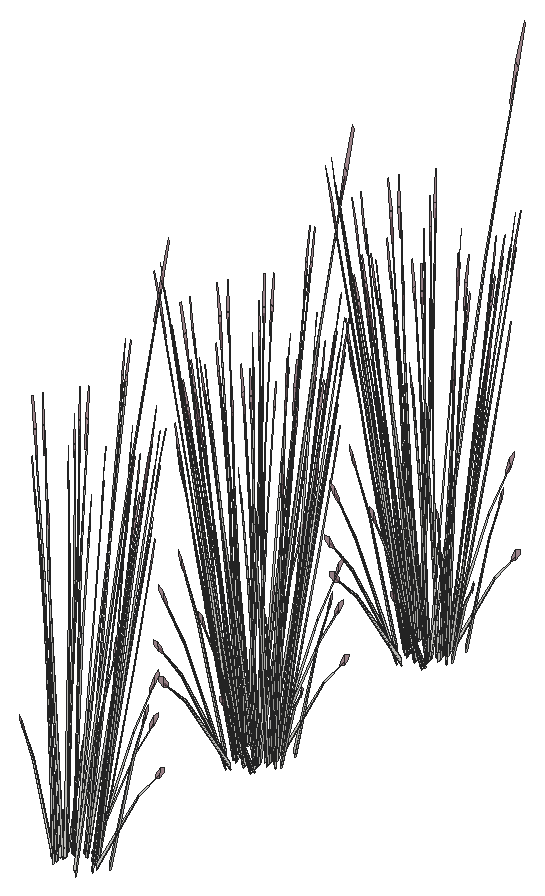
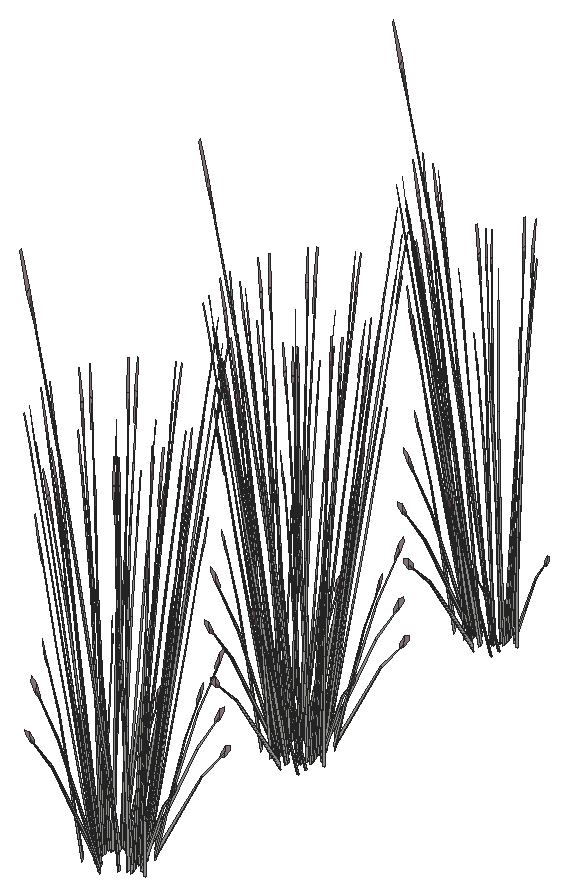
# SketchUp Ruby script. Lengths in inches.
U = 1.inch
M = Sketchup.active_model
def pt(a) = Geom::Point3d.new(a.map { |v| v * U })
def face(e, loops, mat)
  f = e.add_face(loops[0].map { |a| pt(a) })
  loops[1..].each { |l| e.add_face(l.map { |a| pt(a) }).erase! }
  f.material = f.back_material = mat if mat
  f
end
# faces: each face lists its corners as indices into pts; further lists are holes
def faces(e, pts, list, mat = nil) = list.each { |f| face(e, (f[0].is_a?(Array) ? f : [f]).map { |l| l.map { |i| pts[i] } }, mat) }
# xy, xz, yz: faces in a plane at the given z, y or x. An outline is a flat list of corners, or four numbers for a rectangle; further outlines are holes
def ring(l) = l.size == 4 ? [[l[0], l[1]], [l[2], l[1]], [l[2], l[3]], [l[0], l[3]]] : l.each_slice(2).to_a
def flat(e, list, mat, &to3) = list.each { |f| face(e, (f[0].is_a?(Array) ? f : [f]).map { |l| ring(l).map { |u, v| to3.(u, v) } }, mat) }
def xy(e, z, list, mat = nil) = flat(e, list, mat) { |x, y| [x, y, z] }
def xz(e, y, list, mat = nil) = flat(e, list, mat) { |x, z| [x, y, z] }
def yz(e, x, list, mat = nil) = flat(e, list, mat) { |y, z| [x, y, z] }
def lines(e, pts, list) = list.each { |a, b| e.add_line(pt(pts[a]), pt(pts[b])) }
# prism: a flat outline (further loops are holes) pulled along v
def prism(e, loops, v, mat = nil)
  f = face(e, loops, mat); d = Geom::Vector3d.new(v.map { |x| x * U })
  f.pushpull(f.normal.samedirection?(d) ? d.length : -d.length)
end
def box(e, o, s, mat = nil) = prism(e, [[o, [o[0] + s[0], o[1], o[2]], [o[0] + s[0], o[1] + s[1], o[2]], [o[0], o[1] + s[1], o[2]]]], [0, 0, s[2]], mat)
def at(x, y, z, deg = 0) = Geom::Transformation.translation(pt([x, y, z])) * Geom::Transformation.rotation(ORIGIN, Z_AXIS, deg.degrees)
def axes(o, x, y, z) = Geom::Transformation.new([*x, 0, *y, 0, *z, 0, *pt(o).to_a, 1])
def part(name) = M.definitions.add(name)
# library, detail: a bought-in or finely detailed component or shape, given as its bounding box
def library(name, o, s) = part(name).tap { |d| box(d.entities, o, s) }
def detail(e, o, s) = box(e.add_group.entities, o, s)
def put(e, d, t, mat = nil) = e.add_instance(d, t).tap { |i| i.material = mat if mat }
def group(e, t, mat = nil) = e.add_group.tap { |g| g.transformation = t; g.material = mat if mat }.entities
root = M.entities
M.materials.add("LightPink_Translucent").color = [144, 107, 117]
M.materials["LightPink_Translucent"].alpha = 0.75
c1 = part("blade")
p = [[2.15,0.21,22],[0,0.17,0],[0.09,0.45,0],[2.18,0.31,22],[2.29,0.31,22],[0.38,0.45,0],
  [2.48,0.24,33],[2.49,0.24,33],[2.48,0.22,33]]
faces(c1.entities,p,[[0,1,2,3],[4,5,2,3],[6,3,4,7],[8,0,3,6]])
c2 = part("seeds")
p = [[0.3,-0.1,1.38],[-0.01,-0.03,1.59],[-0.01,-0.03,0.03],[0.14,-0.07,-0.07],[0.29,-0.03,3],[0.15,0.01,3.11]]
faces(c2.entities,p,[[0,1,2,3],[1,0,4,5]],"LightPink_Translucent")
c3 = part("blade with seeds")
put(c3.entities,c1,at(0,0,0))
put(c3.entities,c2,axes([2.4,0.25,30.99],[1.5799,-0.05474,1.17369],[-0.12525,1.92788,0.29478],[-0.07173,-0.02425,1.56792]))
put(root,c3,axes([403.71,539.25,4.73],[-0.09971,0.42522,0.48003],[-0.32782,-0.1454,0.3958],[0.12892,-0.02555,0.9933]))
put(root,c3,axes([400.64,538.56,5.05],[0.29332,0.1301,0.35414],[-0.08555,0.37955,-0.4572],[-0.11809,0.0348,0.87481]))
put(root,c3,axes([404.3,540.63,4.71],[-0.03191,-0.04083,1.77383],[0.06981,-0.43764,-0.16761],[0.12571,-0.02796,0.31391]))
put(root,c3,axes([400.14,538.85,4.72],[-0.05763,0.06055,1.74944],[0.0049,0.44239,-0.27667],[-0.13211,0.05753,0.14031]))
put(root,c3,axes([400.51,538.43,5.03],[0.17758,0.42229,-0.1216],[-0.31518,0.20752,-0.67495],[-0.13282,0.05572,1.02557]))
put(root,c3,axes([403.19,540.25,5.03],[0.0189,-0.47427,-0.1216],[0.35781,0.01296,-0.67495],[0.13781,0.03295,1.02557]))
put(root,c3,axes([403.14,540.07,5.05],[-0.20082,-0.29199,0.35414],[0.2293,-0.2764,-0.4572],[0.1165,0.04206,0.87481]))
put(root,c3,axes([403.5,539.97,4.72],[0.07571,-0.00789,1.74944],[0.20767,-0.36231,-0.27667],[0.13467,0.04783,0.14031]))
put(root,c3,axes([400.47,539.61,4.73],[-0.08753,-0.42921,0.48003],[0.34336,-0.07449,0.3958],[-0.1012,0.10094,0.9933]))
put(root,c3,axes([400.41,539.53,4.73],[-0.2423,-0.19613,0.0643],[0.14107,-0.2793,0.50621],[-0.07768,0.0903,0.77189]))
put(root,c3,axes([400.6875,539.47,5.05],[0.30722,-0.06665,0.35414],[0.08112,0.381,-0.4572],[-0.08804,0.10234,0.87481]))
put(root,c3,axes([399.5,539.3,4.71],[0.04504,0.01251,1.77383],[0.13934,0.41205,-0.16761],[-0.0922,0.10815,0.31391]))
put(root,c3,axes([403.32,540.33,4.73],[-0.01777,0.35463,0.0643],[-0.26836,-0.00972,0.50621],[0.1028,0.03711,0.77189]))
put(root,c3,axes([403.34,540.22,4.73],[-0.26024,0.30729,0.48003],[-0.22444,-0.32634,0.3958],[0.1221,0.05668,0.9933]))
put(root,c3,axes([399.99,540.55,5.65],[0.31145,0.12449,-0.06488],[-0.0958,0.38314,-0.29416],[-0.05094,0.05817,0.97024]))
put(root,c3,axes([402.52,540.57,5.05],[-0.05451,-0.37564,0.35414],[0.31161,-0.09919,-0.4572],[0.0837,0.10765,0.87481]))
put(root,c3,axes([402.72,538.41,4.47],[-0.30498,-0.24231,1.38283],[0.32203,-0.37727,0.59665],[0.0984,0.22736,1.33663]))
put(root,c3,axes([400.53,539.4375,5.03],[0.32648,0.25715,-0.1216],[-0.18809,0.3724,-0.67495],[-0.09224,0.12945,1.02557]))
put(root,c3,axes([402.49,540.77,5.03],[0.21031,-0.39918,-0.1216],[0.30457,0.22997,-0.67495],[0.10587,0.11278,1.02557]))
put(root,c3,axes([401.1,540.23,5.05],[0.23881,-0.24554,0.35414],[0.22606,0.28036,-0.4572],[-0.0344,0.14245,0.87481]))
put(root,c3,axes([402.21,541.1,4.71],[0.00104,-0.05646,1.77383],[0.30246,-0.2491,-0.16761],[0.10506,0.08891,0.31391]))
put(root,c3,axes([400.88,540.45,4.73],[-0.29004,-0.02173,0.0643],[0.00795,-0.32812,0.50621],[-0.03035,0.12569,0.77189]))
put(root,c3,axes([400.98,540.48,4.73],[-0.25132,-0.3182,0.48003],[0.2669,-0.27442,0.3958],[-0.04636,0.14929,0.9933]))
put(root,c3,axes([401.77,540.63,5.05],[0.1064,-0.35863,0.35414],[0.31043,0.1046,-0.4572],[0.02846,0.14439,0.87481]))
put(root,c3,axes([402.56,540.91,4.73],[-0.16041,0.29625,0.0643],[-0.22843,-0.17248,0.50621],[0.07385,0.09498,0.77189]))
put(root,c3,axes([402.1875,541.91,5.65],[0.2439,-0.26754,-0.06488],[0.22348,0.29302,-0.29416],[0.01573,0.08303,0.97024]))
put(root,c3,axes([402.63,540.83,4.73],[-0.35104,0.10702,0.48003],[-0.06092,-0.41983,0.3958],[0.08256,0.12373,0.9933]))
put(root,c3,axes([401.67,540.96,4.73],[-0.26007,0.1585,0.0643],[-0.12729,-0.28902,0.50621],[0.02512,0.1274,0.77189]))
put(root,c3,axes([400.15,540.51,4.72],[-0.00877,0.09229,1.74944],[0.24897,0.32105,-0.27667],[-0.06518,0.15182,0.14031]))
put(root,c3,axes([400.95,540.3,5.4],[0.3879,0.02311,-0.13498],[-0.0106,0.43749,-0.74919],[-0.02694,0.1685,1.13838]))
put(root,c3,axes([401.67,540.78,5.03],[0.34538,-0.21713,-0.1216],[0.16972,0.38536,-0.67495],[0.04557,0.16239,1.02557]))
put(root,c3,axes([401.77,540.93,5.0625],[-0.34777,-0.12192,0.53283],[0.11892,-0.40083,0.43934],[0.0209,0.15763,1.10256]))
put(root,c3,axes([400.125,541.45,4.71],[0.04004,-0.02816,1.77383],[0.33095,0.18728,-0.16761],[-0.00778,0.15594,0.31391]))
put(root,c3,axes([401.58,541.65,4.72],[0.04474,0.0751,1.74944],[0.36104,0.0295,-0.27667],[0.03631,0.16562,0.14031]))
put(root,c3,axes([401.89,557.86,4.72],[-0.05398,-0.06539,1.74944],[-0.36026,0.04145,-0.27667],[-0.0575,-0.15639,0.14031]))
put(root,c3,axes([403.51,558.66,4.72],[-0.00341,-0.09282,1.74944],[-0.28775,-0.26825,-0.27667],[0.04449,-0.16261,0.14031]))
put(root,c3,axes([403.43,558.33,4.71],[-0.03584,0.03562,1.77383],[-0.35118,-0.12018,-0.16761],[-0.01271,-0.15545,0.31391]))
put(root,c3,axes([401.52,557.64,4.71],[-0.00658,0.0559,1.77383],[-0.32474,0.20287,-0.16761],[-0.09556,-0.1037,0.31391]))
put(root,c3,axes([401.45,558.64,5.09],[0.39316,-0.11987,0.53763],[0.06823,0.47021,0.4433],[-0.09247,-0.13858,1.11249]))
put(root,c3,axes([402.34,558.72,4.73],[0.34777,0.12192,0.48003],[-0.11892,0.40083,0.3958],[-0.0209,-0.15763,0.9933]))
put(root,c3,axes([402.4375,558.87,5.03],[-0.34538,0.21713,-0.1216],[-0.16972,-0.38536,-0.67495],[-0.04557,-0.16239,1.02557]))
put(root,c3,axes([403.15,559.36,5.03],[-0.3879,-0.02311,-0.1216],[0.0106,-0.43749,-0.67495],[0.02694,-0.1685,1.02557]))
put(root,c3,axes([402.43,558.69,4.73],[0.26007,-0.1585,0.0643],[0.12729,0.28902,0.50621],[-0.02512,-0.1274,0.77189]))
put(root,c3,axes([401.54,558.74,4.73],[0.16041,-0.29625,0.0643],[0.22843,0.17248,0.50621],[-0.07385,-0.09498,0.77189]))
put(root,c3,axes([402.33,559.02,5.05],[-0.1064,0.35863,0.35414],[-0.31043,-0.1046,-0.4572],[-0.02846,-0.14439,0.87481]))
put(root,c3,axes([403.125,559.17,4.73],[0.25132,0.3182,0.48003],[-0.2669,0.27442,0.3958],[0.04636,-0.14929,0.9933]))
put(root,c3,axes([401.61,558.71,5.43],[-0.23555,0.44708,-0.13619],[-0.34112,-0.25757,-0.75594],[-0.11858,-0.12631,1.14864]))
put(root,c3,axes([403.22,559.2,4.73],[0.29004,0.02173,0.0643],[-0.00795,0.32812,0.50621],[0.03035,-0.12569,0.77189]))
put(root,c3,axes([403,559.42,5.05],[-0.23881,0.24554,0.35414],[-0.22606,-0.28036,-0.4572],[0.0344,-0.14245,0.87481]))
put(root,c3,axes([400.71,558.58,4.72],[-0.07594,-0.00329,1.74944],[-0.24177,0.32918,-0.27667],[-0.129,-0.06726,0.14031]))
put(root,c3,axes([403.58,560.22,5.03],[-0.32648,-0.25715,-0.1216],[0.18809,-0.3724,-0.67495],[0.09224,-0.12945,1.02557]))
put(root,c3,axes([401.59,559.08,5.05],[0.05451,0.37564,0.35414],[-0.31161,0.09919,-0.4572],[-0.0837,-0.10765,0.87481]))
put(root,c3,axes([400.65,559.32,5.09],[0.29147,-0.34417,0.53763],[0.25138,0.3655,0.4433],[-0.13675,-0.06349,1.11249]))
put(root,c3,axes([404.38,560.11,4.71],[-0.0461,-0.00354,1.77383],[-0.19143,-0.37951,-0.16761],[0.07688,-0.12478,0.31391]))
put(root,c3,axes([400.78,559.32,4.73],[0.01777,-0.35463,0.0643],[0.26836,0.00972,0.50621],[-0.1028,-0.03711,0.77189]))
put(root,c3,axes([403.42,560.18,5.05],[-0.30722,0.06665,0.35414],[-0.08112,-0.381,-0.4572],[0.08804,-0.10234,0.87481]))
put(root,c3,axes([403.7,560.12,4.73],[0.2423,0.19613,0.0643],[-0.14107,0.2793,0.50621],[0.07768,-0.0903,0.77189]))
put(root,c3,axes([403.63,560.04,4.73],[0.08753,0.42921,0.48003],[-0.34336,0.07449,0.3958],[0.1012,-0.10094,0.9933]))
put(root,c3,axes([404.55,560.56,4.72],[0.04898,-0.07104,1.74944],[-0.06269,-0.43574,-0.27667],[0.12289,-0.08262,0.14031]))
put(root,c3,axes([400.42,558.86,4.71],[0.02617,0.04654,1.77383],[-0.12614,0.41836,-0.16761],[-0.12775,0.00303,0.31391]))
put(root,c3,axes([400.97,559.59,5.05],[0.20082,0.29199,0.35414],[-0.2293,0.2764,-0.4572],[-0.1165,-0.04206,0.87481]))
put(root,c3,axes([400.91,559.4,5.03],[-0.0189,0.47427,-0.1216],[-0.35781,-0.01296,-0.67495],[-0.13781,-0.03295,1.02557]))
put(root,c3,axes([403.59,561.22,5.03],[-0.17758,-0.42229,-0.1216],[0.31518,-0.20752,-0.67495],[0.13282,-0.05572,1.02557]))
put(root,c3,axes([403.47,561.09,5.05],[-0.29332,-0.1301,0.35414],[0.08555,-0.37955,-0.4572],[0.11809,-0.0348,0.87481]))
put(root,c3,axes([400.4,560.4,4.73],[0.09971,-0.42522,0.48003],[0.32782,0.1454,0.3958],[-0.12892,0.02555,0.9933]))
put(root,c3,axes([400.37,560.29,4.73],[-0.12963,-0.31798,0.0643],[0.23638,-0.15564,0.50621],[-0.1042,0.03071,0.77189]))
put(root,c3,axes([403.73,561.21,4.73],[0.12963,0.31798,0.0643],[-0.23638,0.15564,0.50621],[0.1042,-0.03071,0.77189]))
put(root,c3,axes([403.71,561.1,4.73],[-0.09971,0.42522,0.48003],[-0.32782,-0.1454,0.3958],[0.12892,-0.02555,0.9933]))
put(root,c3,axes([400.64,560.4,5.05],[0.29332,0.1301,0.35414],[-0.08555,0.37955,-0.4572],[-0.11809,0.0348,0.87481]))
put(root,c3,axes([404.3,562.47,4.71],[-0.03191,-0.04083,1.77383],[0.06981,-0.43764,-0.16761],[0.12571,-0.02796,0.31391]))
put(root,c3,axes([400.14,560.7,4.72],[-0.05763,0.06055,1.74944],[0.0049,0.44239,-0.27667],[-0.13211,0.05753,0.14031]))
put(root,c3,axes([400.51,560.28,5.03],[0.17758,0.42229,-0.1216],[-0.31518,0.20752,-0.67495],[-0.13282,0.05572,1.02557]))
put(root,c3,axes([403.19,562.1,5.03],[0.0189,-0.47427,-0.1216],[0.35781,0.01296,-0.67495],[0.13781,0.03295,1.02557]))
put(root,c3,axes([403.14,561.91,5.05],[-0.20082,-0.29199,0.35414],[0.2293,-0.2764,-0.4572],[0.1165,0.04206,0.87481]))
put(root,c3,axes([403.5,561.8125,4.72],[0.07571,-0.00789,1.74944],[0.20767,-0.36231,-0.27667],[0.13467,0.04783,0.14031]))
put(root,c3,axes([400.47,561.46,4.73],[-0.08753,-0.42921,0.48003],[0.34336,-0.07449,0.3958],[-0.1012,0.10094,0.9933]))
put(root,c3,axes([400.41,561.375,4.73],[-0.2423,-0.19613,0.0643],[0.14107,-0.2793,0.50621],[-0.07768,0.0903,0.77189]))
put(root,c3,axes([400.6875,561.32,5.05],[0.30722,-0.06665,0.35414],[0.08112,0.381,-0.4572],[-0.08804,0.10234,0.87481]))
put(root,c3,axes([399.5,561.15,4.71],[0.04504,0.01251,1.77383],[0.13934,0.41205,-0.16761],[-0.0922,0.10815,0.31391]))
put(root,c3,axes([403.32,562.18,4.73],[-0.01777,0.35463,0.0643],[-0.26836,-0.00972,0.50621],[0.1028,0.03711,0.77189]))
put(root,c3,axes([403.34,562.0625,4.73],[-0.26024,0.30729,0.48003],[-0.22444,-0.32634,0.3958],[0.1221,0.05668,0.9933]))
put(root,c3,axes([399.99,562.4,5.65],[0.31145,0.12449,-0.06488],[-0.0958,0.38314,-0.29416],[-0.05094,0.05817,0.97024]))
put(root,c3,axes([402.52,562.42,5.05],[-0.05451,-0.37564,0.35414],[0.31161,-0.09919,-0.4572],[0.0837,0.10765,0.87481]))
put(root,c3,axes([402.72,560.26,4.47],[-0.30498,-0.24231,1.38283],[0.32203,-0.37727,0.59665],[0.0984,0.22736,1.33663]))
put(root,c3,axes([400.53,561.28,5.03],[0.32648,0.25715,-0.1216],[-0.18809,0.3724,-0.67495],[-0.09224,0.12945,1.02557]))
put(root,c3,axes([402.49,562.61,5.03],[0.21031,-0.39918,-0.1216],[0.30457,0.22997,-0.67495],[0.10587,0.11278,1.02557]))
put(root,c3,axes([401.1,562.07,5.05],[0.23881,-0.24554,0.35414],[0.22606,0.28036,-0.4572],[-0.0344,0.14245,0.87481]))
put(root,c3,axes([402.21,562.94,4.71],[0.00104,-0.05646,1.77383],[0.30246,-0.2491,-0.16761],[0.10506,0.08891,0.31391]))
put(root,c3,axes([400.88,562.3,4.73],[-0.29004,-0.02173,0.0643],[0.00795,-0.32812,0.50621],[-0.03035,0.12569,0.77189]))
put(root,c3,axes([400.98,562.33,4.73],[-0.25132,-0.3182,0.48003],[0.2669,-0.27442,0.3958],[-0.04636,0.14929,0.9933]))
put(root,c3,axes([401.77,562.48,5.05],[0.1064,-0.35863,0.35414],[0.31043,0.1046,-0.4572],[0.02846,0.14439,0.87481]))
put(root,c3,axes([402.56,562.76,4.73],[-0.16041,0.29625,0.0643],[-0.22843,-0.17248,0.50621],[0.07385,0.09498,0.77189]))
put(root,c3,axes([402.1875,563.76,5.65],[0.2439,-0.26754,-0.06488],[0.22348,0.29302,-0.29416],[0.01573,0.08303,0.97024]))
put(root,c3,axes([402.63,562.68,4.73],[-0.35104,0.10702,0.48003],[-0.06092,-0.41983,0.3958],[0.08256,0.12373,0.9933]))
put(root,c3,axes([401.67,562.8,4.73],[-0.26007,0.1585,0.0643],[-0.12729,-0.28902,0.50621],[0.02512,0.1274,0.77189]))
put(root,c3,axes([400.15,562.35,4.72],[-0.00877,0.09229,1.74944],[0.24897,0.32105,-0.27667],[-0.06518,0.15182,0.14031]))
put(root,c3,axes([400.95,562.14,5.4],[0.3879,0.02311,-0.13498],[-0.0106,0.43749,-0.74919],[-0.02694,0.1685,1.13838]))
put(root,c3,axes([401.67,562.63,5.03],[0.34538,-0.21713,-0.1216],[0.16972,0.38536,-0.67495],[0.04557,0.16239,1.02557]))
put(root,c3,axes([401.77,562.77,5.0625],[-0.34777,-0.12192,0.53283],[0.11892,-0.40083,0.43934],[0.0209,0.15763,1.10256]))
put(root,c3,axes([400.125,563.3,4.71],[0.04004,-0.02816,1.77383],[0.33095,0.18728,-0.16761],[-0.00778,0.15594,0.31391]))
put(root,c3,axes([401.58,563.49,4.72],[0.04474,0.0751,1.74944],[0.36104,0.0295,-0.27667],[0.03631,0.16562,0.14031]))
put(root,c3,axes([401.89,578.125,4.72],[-0.05398,-0.06539,1.74944],[-0.36026,0.04145,-0.27667],[-0.0575,-0.15639,0.14031]))
put(root,c3,axes([403.51,578.93,4.72],[-0.00341,-0.09282,1.74944],[-0.28775,-0.26825,-0.27667],[0.04449,-0.16261,0.14031]))
put(root,c3,axes([403.43,578.59,4.71],[-0.03584,0.03562,1.77383],[-0.35118,-0.12018,-0.16761],[-0.01271,-0.15545,0.31391]))
put(root,c3,axes([401.52,577.91,4.71],[-0.00658,0.0559,1.77383],[-0.32474,0.20287,-0.16761],[-0.09556,-0.1037,0.31391]))
put(root,c3,axes([401.45,578.9,5.09],[0.39316,-0.11987,0.53763],[0.06823,0.47021,0.4433],[-0.09247,-0.13858,1.11249]))
put(root,c3,axes([402.34,578.99,4.73],[0.34777,0.12192,0.48003],[-0.11892,0.40083,0.3958],[-0.0209,-0.15763,0.9933]))
put(root,c3,axes([402.4375,579.14,5.03],[-0.34538,0.21713,-0.1216],[-0.16972,-0.38536,-0.67495],[-0.04557,-0.16239,1.02557]))
put(root,c3,axes([403.15,579.625,5.03],[-0.3879,-0.02311,-0.1216],[0.0106,-0.43749,-0.67495],[0.02694,-0.1685,1.02557]))
put(root,c3,axes([402.43,578.96,4.73],[0.26007,-0.1585,0.0643],[0.12729,0.28902,0.50621],[-0.02512,-0.1274,0.77189]))
put(root,c3,axes([401.54,579.01,4.73],[0.16041,-0.29625,0.0643],[0.22843,0.17248,0.50621],[-0.07385,-0.09498,0.77189]))
put(root,c3,axes([402.33,579.29,5.05],[-0.1064,0.35863,0.35414],[-0.31043,-0.1046,-0.4572],[-0.02846,-0.14439,0.87481]))
put(root,c3,axes([403.125,579.4375,4.73],[0.25132,0.3182,0.48003],[-0.2669,0.27442,0.3958],[0.04636,-0.14929,0.9933]))
put(root,c3,axes([401.61,578.97,5.43],[-0.23555,0.44708,-0.13619],[-0.34112,-0.25757,-0.75594],[-0.11858,-0.12631,1.14864]))
put(root,c3,axes([403.22,579.47,4.73],[0.29004,0.02173,0.0643],[-0.00795,0.32812,0.50621],[0.03035,-0.12569,0.77189]))
put(root,c3,axes([403,579.69,5.05],[-0.23881,0.24554,0.35414],[-0.22606,-0.28036,-0.4572],[0.0344,-0.14245,0.87481]))
put(root,c3,axes([400.71,578.85,4.72],[-0.07594,-0.00329,1.74944],[-0.24177,0.32918,-0.27667],[-0.129,-0.06726,0.14031]))
put(root,c3,axes([403.58,580.48,5.03],[-0.32648,-0.25715,-0.1216],[0.18809,-0.3724,-0.67495],[0.09224,-0.12945,1.02557]))
put(root,c3,axes([401.59,579.35,5.05],[0.05451,0.37564,0.35414],[-0.31161,0.09919,-0.4572],[-0.0837,-0.10765,0.87481]))
put(root,c3,axes([400.65,579.59,5.09],[0.29147,-0.34417,0.53763],[0.25138,0.3655,0.4433],[-0.13675,-0.06349,1.11249]))
put(root,c3,axes([404.38,580.37,4.71],[-0.0461,-0.00354,1.77383],[-0.19143,-0.37951,-0.16761],[0.07688,-0.12478,0.31391]))
put(root,c3,axes([400.78,579.59,4.73],[0.01777,-0.35463,0.0643],[0.26836,0.00972,0.50621],[-0.1028,-0.03711,0.77189]))
put(root,c3,axes([403.42,580.45,5.05],[-0.30722,0.06665,0.35414],[-0.08112,-0.381,-0.4572],[0.08804,-0.10234,0.87481]))
put(root,c3,axes([403.7,580.39,4.73],[0.2423,0.19613,0.0643],[-0.14107,0.2793,0.50621],[0.07768,-0.0903,0.77189]))
put(root,c3,axes([403.63,580.31,4.73],[0.08753,0.42921,0.48003],[-0.34336,0.07449,0.3958],[0.1012,-0.10094,0.9933]))
put(root,c3,axes([404.55,580.83,4.72],[0.04898,-0.07104,1.74944],[-0.06269,-0.43574,-0.27667],[0.12289,-0.08262,0.14031]))
put(root,c3,axes([400.42,579.125,4.71],[0.02617,0.04654,1.77383],[-0.12614,0.41836,-0.16761],[-0.12775,0.00303,0.31391]))
put(root,c3,axes([400.97,579.85,5.05],[0.20082,0.29199,0.35414],[-0.2293,0.2764,-0.4572],[-0.1165,-0.04206,0.87481]))
put(root,c3,axes([400.91,579.67,5.03],[-0.0189,0.47427,-0.1216],[-0.35781,-0.01296,-0.67495],[-0.13781,-0.03295,1.02557]))
put(root,c3,axes([403.59,581.49,5.03],[-0.17758,-0.42229,-0.1216],[0.31518,-0.20752,-0.67495],[0.13282,-0.05572,1.02557]))
put(root,c3,axes([403.47,581.36,5.05],[-0.29332,-0.1301,0.35414],[0.08555,-0.37955,-0.4572],[0.11809,-0.0348,0.87481]))
put(root,c3,axes([400.4,580.67,4.73],[0.09971,-0.42522,0.48003],[0.32782,0.1454,0.3958],[-0.12892,0.02555,0.9933]))
put(root,c3,axes([400.37,580.55,4.73],[-0.12963,-0.31798,0.0643],[0.23638,-0.15564,0.50621],[-0.1042,0.03071,0.77189]))
put(root,c3,axes([403.73,581.48,4.73],[0.12963,0.31798,0.0643],[-0.23638,0.15564,0.50621],[0.1042,-0.03071,0.77189]))
put(root,c3,axes([403.71,581.37,4.73],[-0.09971,0.42522,0.48003],[-0.32782,-0.1454,0.3958],[0.12892,-0.02555,0.9933]))
put(root,c3,axes([400.64,580.67,5.05],[0.29332,0.1301,0.35414],[-0.08555,0.37955,-0.4572],[-0.11809,0.0348,0.87481]))
put(root,c3,axes([404.3,582.74,4.71],[-0.03191,-0.04083,1.77383],[0.06981,-0.43764,-0.16761],[0.12571,-0.02796,0.31391]))
put(root,c3,axes([400.14,580.97,4.72],[-0.05763,0.06055,1.74944],[0.0049,0.44239,-0.27667],[-0.13211,0.05753,0.14031]))
put(root,c3,axes([400.51,580.54,5.03],[0.17758,0.42229,-0.1216],[-0.31518,0.20752,-0.67495],[-0.13282,0.05572,1.02557]))
put(root,c3,axes([403.19,582.37,5.03],[0.0189,-0.47427,-0.1216],[0.35781,0.01296,-0.67495],[0.13781,0.03295,1.02557]))
put(root,c3,axes([403.14,582.18,5.05],[-0.20082,-0.29199,0.35414],[0.2293,-0.2764,-0.4572],[0.1165,0.04206,0.87481]))
put(root,c3,axes([403.5,582.08,4.72],[0.07571,-0.00789,1.74944],[0.20767,-0.36231,-0.27667],[0.13467,0.04783,0.14031]))
put(root,c3,axes([400.47,581.73,4.73],[-0.08753,-0.42921,0.48003],[0.34336,-0.07449,0.3958],[-0.1012,0.10094,0.9933]))
put(root,c3,axes([400.41,581.64,4.73],[-0.2423,-0.19613,0.0643],[0.14107,-0.2793,0.50621],[-0.07768,0.0903,0.77189]))
put(root,c3,axes([400.6875,581.58,5.05],[0.30722,-0.06665,0.35414],[0.08112,0.381,-0.4572],[-0.08804,0.10234,0.87481]))
put(root,c3,axes([399.5,581.41,4.71],[0.04504,0.01251,1.77383],[0.13934,0.41205,-0.16761],[-0.0922,0.10815,0.31391]))
put(root,c3,axes([403.32,582.44,4.73],[-0.01777,0.35463,0.0643],[-0.26836,-0.00972,0.50621],[0.1028,0.03711,0.77189]))
put(root,c3,axes([403.34,582.33,4.73],[-0.26024,0.30729,0.48003],[-0.22444,-0.32634,0.3958],[0.1221,0.05668,0.9933]))
put(root,c3,axes([399.99,582.66,5.65],[0.31145,0.12449,-0.06488],[-0.0958,0.38314,-0.29416],[-0.05094,0.05817,0.97024]))
put(root,c3,axes([402.52,582.6875,5.05],[-0.05451,-0.37564,0.35414],[0.31161,-0.09919,-0.4572],[0.0837,0.10765,0.87481]))
put(root,c3,axes([402.72,580.53,4.47],[-0.30498,-0.24231,1.38283],[0.32203,-0.37727,0.59665],[0.0984,0.22736,1.33663]))
put(root,c3,axes([400.53,581.55,5.03],[0.32648,0.25715,-0.1216],[-0.18809,0.3724,-0.67495],[-0.09224,0.12945,1.02557]))
put(root,c3,axes([402.49,582.88,5.03],[0.21031,-0.39918,-0.1216],[0.30457,0.22997,-0.67495],[0.10587,0.11278,1.02557]))
put(root,c3,axes([401.1,582.34,5.05],[0.23881,-0.24554,0.35414],[0.22606,0.28036,-0.4572],[-0.0344,0.14245,0.87481]))
put(root,c3,axes([402.21,583.21,4.71],[0.00104,-0.05646,1.77383],[0.30246,-0.2491,-0.16761],[0.10506,0.08891,0.31391]))
